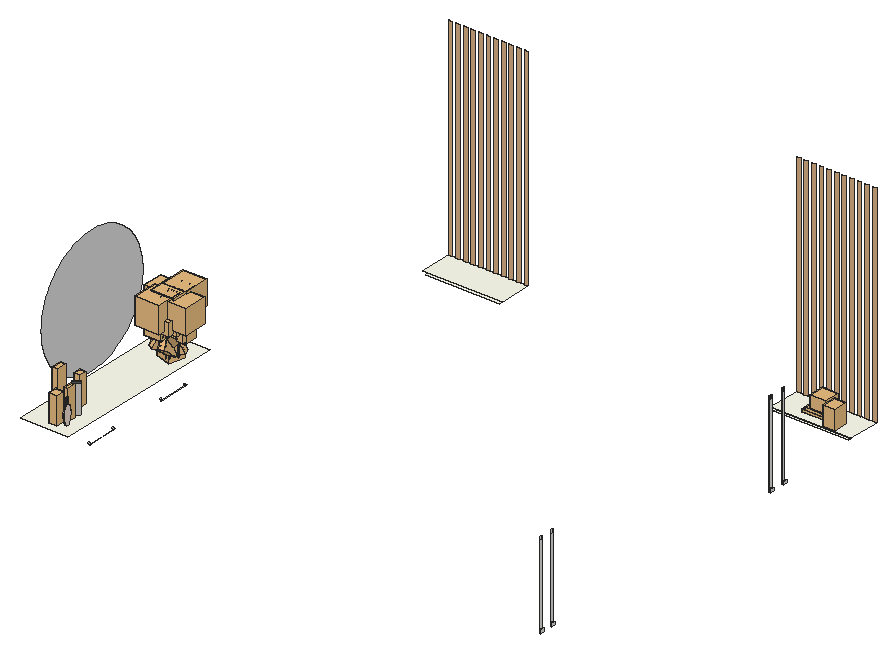
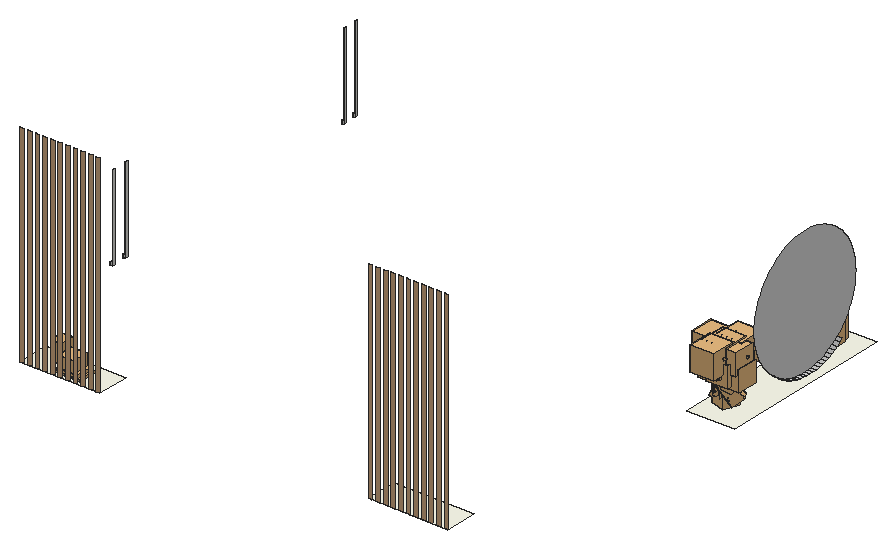
# SketchUp Ruby script. Lengths in inches.
U = 1.inch
M = Sketchup.active_model
def pt(a) = Geom::Point3d.new(a.map { |v| v * U })
def face(e, loops, mat)
  f = e.add_face(loops[0].map { |a| pt(a) })
  loops[1..].each { |l| e.add_face(l.map { |a| pt(a) }).erase! }
  f.material = f.back_material = mat if mat
  f
end
# faces: each face lists its corners as indices into pts; further lists are holes
def faces(e, pts, list, mat = nil) = list.each { |f| face(e, (f[0].is_a?(Array) ? f : [f]).map { |l| l.map { |i| pts[i] } }, mat) }
# xy, xz, yz: faces in a plane at the given z, y or x. An outline is a flat list of corners, or four numbers for a rectangle; further outlines are holes
def ring(l) = l.size == 4 ? [[l[0], l[1]], [l[2], l[1]], [l[2], l[3]], [l[0], l[3]]] : l.each_slice(2).to_a
def flat(e, list, mat, &to3) = list.each { |f| face(e, (f[0].is_a?(Array) ? f : [f]).map { |l| ring(l).map { |u, v| to3.(u, v) } }, mat) }
def xy(e, z, list, mat = nil) = flat(e, list, mat) { |x, y| [x, y, z] }
def xz(e, y, list, mat = nil) = flat(e, list, mat) { |x, z| [x, y, z] }
def yz(e, x, list, mat = nil) = flat(e, list, mat) { |y, z| [x, y, z] }
def lines(e, pts, list) = list.each { |a, b| e.add_line(pt(pts[a]), pt(pts[b])) }
# prism: a flat outline (further loops are holes) pulled along v
def prism(e, loops, v, mat = nil)
  f = face(e, loops, mat); d = Geom::Vector3d.new(v.map { |x| x * U })
  f.pushpull(f.normal.samedirection?(d) ? d.length : -d.length)
end
def box(e, o, s, mat = nil) = prism(e, [[o, [o[0] + s[0], o[1], o[2]], [o[0] + s[0], o[1] + s[1], o[2]], [o[0], o[1] + s[1], o[2]]]], [0, 0, s[2]], mat)
def at(x, y, z, deg = 0) = Geom::Transformation.translation(pt([x, y, z])) * Geom::Transformation.rotation(ORIGIN, Z_AXIS, deg.degrees)
def axes(o, x, y, z) = Geom::Transformation.new([*x, 0, *y, 0, *z, 0, *pt(o).to_a, 1])
def part(name) = M.definitions.add(name)
# library, detail: a bought-in or finely detailed component or shape, given as its bounding box
def library(name, o, s) = part(name).tap { |d| box(d.entities, o, s) }
def detail(e, o, s) = box(e.add_group.entities, o, s)
def put(e, d, t, mat = nil) = e.add_instance(d, t).tap { |i| i.material = mat if mat }
def group(e, t, mat = nil) = e.add_group.tap { |g| g.transformation = t; g.material = mat if mat }.entities
root = M.entities
M.materials.add("Guerlain-Terracotta-Le-parfum1").color = [235, 217, 205]
M.materials.add("Material \#1").color = [0, 0, 0]
M.materials["Material \#1"].alpha = 0.02
M.materials.add("Material \#2").color = [190, 173, 82]
M.materials.add("[0053_Ivory]").color = [255, 255, 240]
M.materials.add("[0135_DarkGray]").color = [81, 81, 81]
M.materials.add("[Formica Laminate Light]").color = [219, 178, 137]
M.materials.add("[Mirror 02]").color = [216, 216, 216]
M.materials.add("parfumlegacycristianoronaldo").color = [199, 196, 192]
M.materials.add("stebel1").color = [28, 33, 12]
M.materials.add("steklo zelenkovatoie1").color = [255, 255, 255]
M.materials["steklo zelenkovatoie1"].alpha = 0.01
c1 = library("_2_Bo6",[964.11,-137.96,0],[33.44,269.06,364.17])
c2 = library("Potted succulent",[-0.0625,-0.27,0],[4.39,5.31,7.09])
c3 = library("_2_Books_",[998.35,-139.66,0],[33.41,270.76,308.82])
c4 = library("Potted succulent \#1",[-0.84,-0.93,0],[5.95,6.01,4.45])
c5 = library("3DGeom~1_Defintion",[-52.13,-413.8,-261.9],[525.02,1000,523.8])
c6 = library("3DGeom~2_Defintion",[-50.59,-505.34,-385.42],[772.63,1000,770.84])
c7 = library("3DGeom~3_Defintion",[-29.0625,-449.47,-46.19],[316.66,1000,422.96])
c8 = library("3DGeom~4_Defintion",[-108.73,-466.24,-10.56],[206.74,1000,21.12])
c9 = library("3DGeom~24_Defintion",[-29.43,-617.96,-68.09],[452.88,1000,135.79])
c10 = library("3DGeom~25_Defintion",[-610.43,-341.49,-497.01],[982.35,1000,969.41])
c11 = library("3DGeom~26_Defintion",[-154.21,-582.64,-13.2],[230.85,1000,89.07])
c12 = library("3DGeom~46_Defintion",[-99.32,-628.8,-45.04],[163.52,1000,86.15])
c13 = library("3DGeom~47_Defintion",[-610.43,-341.49,-497.01],[982.35,1000,969.41])
c14 = library("3DGeom~67_Defintion",[-119.83,-464.72,-82.11],[221.96,1000,101.36])
c15 = library("3DGeom~68_Defintion",[-87.7,-569.68,-8.51],[166.72,1000,17.02])
c16 = library("3DGeom~88_Defintion",[-29.05,-445.66,-46.32],[158.62,1000,383.8])
c17 = library("3DGeom~108_Defintion",[-29.05,-445.66,-46.32],[158.62,1000,383.8])
c18 = library("3DGeom~128_Defintion",[-59.54,-603.37,-20.8],[132.36,1000,205.61])
c19 = library("3DGeom~210_Defintion",[-52.61,-408.84,-35.61],[338.09,1000,556.23])
c20 = library("3DGeom~148_Defintion",[51.2,-373.87,-225.05],[965.37,1000,237.2])
c21 = library("3DGeom~168_Defintion",[-240.01,-591.63,-7.88],[312.88,1000,313.07])
c22 = library("3DGeom~188_Defintion",[-38.1,-581.48,-8.09],[235.64,1000,465.37])
c23 = library("3DGeom~208_Defintion",[-31.71,-599.5,-29.35],[299.97,1000,62.63])
c24 = library("3DGeom~209_Defintion",[-610.43,-341.49,-497.01],[982.35,1000,969.41])
c25 = library("3DGeom~230_Defintion",[-52.27,-610.5,-175.11],[119.82,1000,194.62])
c26 = library("3DGeom~231_Defintion",[-610.43,-341.49,-497.01],[982.35,1000,969.41])
c27 = library("Group256\#1",[-71.58,-56.43,-7.72],[73.72,80.59,73.34])
c28 = library("Group263\#1",[-46.97,-31.33,7.1875],[18.81,31.79,41.38])
c29 = library("Group287\#1",[-50.75,-46.82,27.36],[89.41,99.07,85.64])
c30 = library("Group294\#1",[-14.22,-12.09,43.13],[18.22,30.92,53.79])
c31 = library("Group317\#1",[-1.3,-52.25,9.83],[15.89,17.75,44.41])
c32 = library("Group337\#1",[-31.87,-82.17,2.6],[77.56,78.87,47.75])
c33 = library("Group347\#1",[-4.2,-64.59,17.37],[101.32,89.76,91.67])
c34 = library("Group354\#1",[24.67,-31.86,36.01],[41.21,18.58,51.73])
c35 = library("Group376\#1",[-63.84,-14.97,-16.9],[80.46,73.53,76.87])
c36 = library("Group383\#1",[-36.625,8.77,7.86],[25.4,35.84,34.54])
c37 = library("Group405\#1",[-23.14,-24.51,-17.79],[74.54,78.39,80.19])
c38 = library("Group412\#1",[-0.27,0.9375,4.5],[35.66,26.25,34.25])
c39 = library("Group434\#1",[-64.79,-104.42,13.66],[92.35,97.65,97.85])
c40 = library("Group441\#1",[-31.23,-78.39,39.84],[22.43,44.95,44.17])
c41 = library("Group463\#1",[-31.71,-70.81,-2.87],[18.58,35.57,19.28])
c42 = library("Group483\#1",[-53.17,-75.45,-26.9375],[66.59,51.19,65.74])
c43 = library("Group492\#1",[-47.04,8.92,24.48],[89.7,95.5,90.68])
c44 = library("Group499\#1",[-12.74,38.04,47.38],[22.44,43.15,45.66])
c45 = library("Group521\#1",[-89.52,-29.26,29.33],[79.87,78.2,80.19])
c46 = library("Group528\#1",[-65.95,-0.45,51.63],[35.33,26.88,34.25])
c47 = library("Group552\#1",[-97.12,-35.39,-24.56],[60.39,79.79,77.7])
c48 = library("Group559\#1",[-90.25,-4.6,5.7],[42.56,22.1,20.27])
c49 = library("Group582\#1",[26.01,-59.49,-2.98],[35.51,41.53,26.85])
c50 = library("Group583\#1",[22.86,-47.74,0.4375],[40.62,39.02,47.67])
c51 = library("Group584\#1",[29.99,-24.89,-5.59],[36.3,43.55,36.22])
c52 = library("Group585\#1",[29.89,-48.04,-26.1],[42.74,35.82,45.2])
c53 = library("Group586\#1",[23.8,-29.02,1.04],[40.9,33.88,46.12])
c54 = library("Group587\#1",[32.33,-33.47,-29.58],[46.05,42.8,51.3])
c55 = library("Group589\#1",[32.61,-23.03,5.86],[38.87,7.41,11.92])
c56 = library("Group592\#1",[31.95,-24.5625,6.27],[41.61,5.99,14.68])
c57 = library("Group595\#1",[31.72,-30.92,5.77],[35.66,11.54,12.18])
c58 = library("Group598\#1",[32.89,-27.72,3.5],[41.82,8.31,12.73])
c59 = library("Group601\#1",[32.85,-23.81,2.26],[39.48,5.21,12.87])
c60 = library("Group604\#1",[32.97,-23.7,0.68],[37.46,10.79,14.46])
c61 = library("Group607\#1",[32.41,-24.57,4.01],[32.05,7.19,11.83])
c62 = part("Group250\#1")
put(c62.entities,c5,axes([-27.93,0.85,-67.89],[0.10942,-0.0328,0],[0,0,0.11423],[-0.0328,-0.10942,0]),"steklo zelenkovatoie1")
put(c62.entities,c6,axes([-27.93,0.85,-67.89],[0.06787,-0.02034,0],[0,0,0.07086],[-0.02034,-0.06787,0]),"Material \#1")
put(c62.entities,c7,axes([-15.1,-12.46,-31.32],[0.07432,0.06349,-0.05506],[0.07739,-0.02306,0.07788],[0.03275,-0.08957,-0.05907]),"stebel1")
put(c62.entities,c8,axes([-26.86,2.88,-49.92],[-0.05357,-0.102,0],[0,0,0.11521],[-0.102,0.05357,0]),"stebel1")
put(c62.entities,c9,axes([-11.34,-17.02,20.09],[-0.0063,0.12632,-0.10549],[-0.04747,0.09969,0.1222],[0.15758,0.03508,0.03259]),"stebel1")
put(c62.entities,c10,axes([-40.61,43.2,69.56],[-0.00654,0.00012,-0.00786],[-0.00561,-0.00724,0.00455],[-0.02646,0.03467,0.02255]),"Material \#2")
put(c62.entities,c11,axes([-18,-11.56,-13.53],[-0.06678,0.12751,0.0315],[0.04218,-0.01264,0.14061],[0.12438,0.07274,-0.03077]),"stebel1")
put(c62.entities,c12,axes([8.55,-18.5625,3.57],[0.16197,-0.04855,0],[0,0,0.16909],[-0.04855,-0.16197,0]),"stebel1")
put(c62.entities,c13,axes([25.0625,-17.88,85.16],[0.00739,0.00592,-0.00387],[-0.00618,0.00812,0.00061],[0.01647,0.00912,0.04534]),"Material \#2")
put(c62.entities,c14,axes([1.14,-28.05,-49.92],[0.04622,-0.10645,0],[0,0,0.11606],[-0.10645,-0.04622,0]),"stebel1")
put(c62.entities,c15,axes([22.47,-14.26,-19.22],[0.13689,-0.04103,0],[0,0,0.1429],[-0.04103,-0.13689,0]),"stebel1")
put(c62.entities,c16,axes([-4.88,-15.48,-41.05],[-0.09455,0.05151,-0.02857],[-0.00894,0.04086,0.10325],[0.05822,0.08993,-0.03055]),"stebel1")
put(c62.entities,c17,axes([-27.48,2.8,-44.87],[0.07693,0.07534,-0.02857],[0.04169,-0.00341,0.10325],[0.06895,-0.08199,-0.03055]),"stebel1")
put(c62.entities,c18,axes([3.67,-12.44,-8.08],[0.05195,-0.14507,-0.01714],[-0.05925,-0.03755,0.13826],[-0.13352,-0.03978,-0.06802]),"stebel1")
put(c62.entities,c19,axes([-3.07,-11.58,-26.29],[-0.07643,-0.04955,-0.05131],[-0.06867,0.03078,0.07257],[-0.01929,0.08676,-0.05505]),"stebel1")
put(c62.entities,c20,axes([0.18,9.9375,-12.85],[-0.02749,-0.03127,-0.07245],[-0.02127,-0.07095,0.03868],[-0.07599,0.03116,0.01538]),"stebel1")
put(c62.entities,c21,axes([-29.92,16.96,0.49],[-0.09159,0.11912,0.01982],[0.07962,0.04088,0.12231],[0.09078,0.08433,-0.08728]),"stebel1")
put(c62.entities,c22,axes([-18.25,-21.22,2.26],[-0.13551,0.04489,-0.03788],[-0.0213,0.0512,0.13688],[0.05473,0.13106,-0.0405]),"stebel1")
put(c62.entities,c23,axes([-16.76,7.75,-0.37],[0.12559,0.07073,-0.06232],[0.05784,0.02417,0.14398],[0.07444,-0.13811,-0.00672]),"stebel1")
put(c62.entities,c24,axes([23.22,32.08,68.47],[-0.00082,0.00868,-0.00535],[-0.00922,0.00166,0.00409],[0.02084,0.02475,0.03693]),"Material \#2")
put(c62.entities,c25,axes([-32.65,4.47,-9.81],[-0.14512,0.04201,-0.05532],[-0.05817,-0.00348,0.14997],[0.03797,0.15527,0.01833]),"stebel1")
put(c62.entities,c26,axes([-77.51,1.58,60.26],[-0.00529,-0.00603,-0.00635],[0.00581,-0.00796,0.00273],[-0.03144,-0.01054,0.03621]),"Material \#2")
put(c62.entities,c27,at(0,0,0))
put(c62.entities,c28,at(0,0,0))
put(c62.entities,c29,at(0,0,0))
put(c62.entities,c30,at(0,0,0))
put(c62.entities,c31,at(0,0,0))
put(c62.entities,c32,at(0,0,0))
put(c62.entities,c33,at(0,0,0))
put(c62.entities,c34,at(0,0,0))
put(c62.entities,c35,at(0,0,0))
put(c62.entities,c36,at(0,0,0))
put(c62.entities,c37,at(0,0,0))
put(c62.entities,c38,at(0,0,0))
put(c62.entities,c39,at(0,0,0))
put(c62.entities,c40,at(0,0,0))
put(c62.entities,c41,at(0,0,0))
put(c62.entities,c42,at(0,0,0))
put(c62.entities,c43,at(0,0,0))
put(c62.entities,c44,at(0,0,0))
put(c62.entities,c45,at(0,0,0))
put(c62.entities,c46,at(0,0,0))
put(c62.entities,c47,at(0,0,0))
put(c62.entities,c48,at(0,0,0))
put(c62.entities,c49,at(0,0,0))
put(c62.entities,c50,at(0,0,0))
put(c62.entities,c51,at(0,0,0))
put(c62.entities,c52,at(0,0,0))
put(c62.entities,c53,at(0,0,0))
put(c62.entities,c54,at(0,0,0))
put(c62.entities,c55,at(0,0,0))
put(c62.entities,c56,at(0,0,0))
put(c62.entities,c57,at(0,0,0))
put(c62.entities,c58,at(0,0,0))
put(c62.entities,c59,at(0,0,0))
put(c62.entities,c60,at(0,0,0))
put(c62.entities,c61,at(0,0,0))
xy(root,43.794,[[24.639,44.595,24.875,56.5],[24.639,78.595,24.875,90.5]])
xy(root,45.244,[[39.88,185,68.12,186],[171.88,185,200.12,186]],"[0053_Ivory]")
xy(root,46.244,[[38.88,185,69.12,197],[170.88,185,201.12,197]],"[0053_Ivory]")
xy(root,50.387,[[19.07,39.927,19.63,40.97]],"Guerlain-Terracotta-Le-parfum1")
xy(root,50.387,[[[6,35.11,24,102.422],[19.07,39.927,19.63,40.97]]],"[0053_Ivory]")
xy(root,50.766,[[17.077,45.58,16.024,46.893,18.094,48.815,19.146,47.503]])
xy(root,52.343,[[210,27.045,209.361,27.38,209.125,27.38,209.125,28.052,209.361,28.052,210,28.388],[210,32.232,209.361,32.568,209.125,32.568,209.125,33.239,209.361,33.239,210,33.575],[210,135.92,209.361,136.255,209.125,136.255,209.125,136.927,209.361,136.927,210,137.263],[210,141.92,209.361,142.255,209.125,142.255,209.125,142.927,209.361,142.927,210,143.263]])
xy(root,53.603,[[210,27.045,210,28.388,209.361,28.052,209.361,27.38],[210,32.232,210,33.575,209.361,33.239,209.361,32.568],[210,135.92,210,137.263,209.361,136.927,209.361,136.255],[210,141.92,210,143.263,209.361,142.927,209.361,142.255]])
xy(root,57.471,[[19.045,40.163,19.649,40.792]],"Guerlain-Terracotta-Le-parfum1")
xy(root,57.984,[[19.353,40.0625,19.254,40.077,19.161,40.118,19.082,40.184,19.021,40.269,18.982,40.369,18.969,40.476,18.982,40.583,19.021,40.682,19.082,40.768,19.161,40.833,19.254,40.875,19.353,40.889,19.452,40.875,19.545,40.833,19.624,40.768,19.685,40.682,19.724,40.583,19.737,40.476,19.724,40.369,19.685,40.269,19.624,40.184,19.545,40.118,19.452,40.077]])
xy(root,59.52,[[19.353,40.0625,19.452,40.077,19.545,40.118,19.624,40.184,19.685,40.269,19.724,40.369,19.737,40.476,19.724,40.583,19.685,40.682,19.624,40.768,19.545,40.833,19.452,40.875,19.353,40.889,19.254,40.875,19.161,40.833,19.082,40.768,19.021,40.682,18.982,40.583,18.969,40.476,18.982,40.369,19.021,40.269,19.082,40.184,19.161,40.118,19.254,40.077]],"[0135_DarkGray]")
xy(root,61.174,[[17.077,45.58,19.146,47.503,18.094,48.815,16.024,46.893]],"[0135_DarkGray]")
xz(root,27.38,[[209.125,52.343,209.361,84.893]])
xz(root,28.052,[[209.125,52.343,209.361,84.893]])
xz(root,32.568,[[209.125,52.343,209.361,84.893]])
xz(root,33.239,[[209.125,52.343,209.361,84.893]])
xz(root,40.156,[[19.045,57.429,19.649,57.436],[19.045,57.436,19.649,57.443]],"Guerlain-Terracotta-Le-parfum1")
xz(root,136.255,[[209.125,52.343,209.361,84.893]])
xz(root,136.927,[[209.125,52.343,209.361,84.893]])
xz(root,142.255,[[209.125,52.343,209.361,84.893]])
xz(root,142.927,[[209.125,52.343,209.361,84.893]])
xz(root,197,[[38.88,46.244,40.32,126],[41.76,46.244,43.2,126],[44.64,46.244,46.08,126],[47.52,46.244,48.96,126],[50.4,46.244,51.84,126],
  [53.28,46.244,54.72,126],[56.16,46.244,57.6,126],[59.04,46.244,60.48,126],[61.92,46.244,63.36,126],[64.8,46.244,66.24,126],
  [67.68,46.244,69.12,126],[170.88,46.244,172.32,126],[173.76,46.244,175.2,126],[176.64,46.244,178.08,126],[179.52,46.244,180.96,126],
  [182.4,46.244,183.84,126],[185.28,46.244,186.72,126],[188.16,46.244,189.6,126],[191.04,46.244,192.48,126],[193.92,46.244,195.36,126],
  [196.8,46.244,198.24,126],[199.68,46.244,201.12,126]],"[Formica Laminate Light]")
yz(root,8,[[66.545,53.326,68.052,53.373,69.553,53.515,71.042,53.751,72.513,54.08,73.961,54.5,75.38,55.011,76.763,55.61,78.107,56.294,79.404,57.062,80.651,57.909,81.843,58.833,82.974,59.831,84.04,60.897,85.037,62.028,85.961,63.219,86.808,64.466,87.576,65.764,88.26,67.107,88.859,68.491,89.37,69.909,89.791,71.357,90.119,72.829,90.355,74.318,90.497,75.819,90.545,77.326,90.497,78.833,90.355,80.334,90.119,81.823,89.791,83.294,89.37,84.742,88.859,86.161,88.26,87.545,87.576,88.888,86.808,90.186,85.961,91.433,85.037,92.624,84.04,93.755,82.974,94.821,81.843,95.818,80.651,96.742,79.404,97.59,78.107,98.357,76.763,99.042,75.38,99.64,73.961,100.151,72.513,100.572,71.042,100.901,69.553,101.137,68.052,101.278,66.545,101.326,65.038,101.278,63.537,101.137,62.047,100.901,60.576,100.572,59.128,100.151,57.71,99.64,56.326,99.042,54.982,98.357,53.685,97.59,52.4375,96.742,51.246,95.818,50.115,94.821,49.049,93.755,48.052,92.624,47.128,91.433,46.281,90.186,45.513,88.888,44.829,87.545,44.23,86.161,43.719,84.742,43.299,83.294,42.97,81.823,42.734,80.334,42.592,78.833,42.545,77.326,42.592,75.819,42.734,74.318,42.97,72.829,43.299,71.357,43.719,69.909,44.23,68.491,44.829,67.107,45.513,65.764,46.281,64.466,47.128,63.219,48.052,62.028,49.049,60.897,50.115,59.831,51.246,58.833,52.4375,57.909,53.685,57.062,54.982,56.294,56.326,55.61,57.71,55.011,59.128,54.5,60.576,54.08,62.047,53.751,63.537,53.515,65.038,53.373]],"[Mirror 02]")
yz(root,19.045,[[40.163,57.4,40.161,57.404,40.159,57.41,40.158,57.415,40.156,57.429,40.156,57.443,40.157,57.449,40.158,57.456,40.159,57.462,40.161,57.467,40.163,57.471,40.792,57.471,40.795,57.47,40.798,57.466,40.801,57.461,40.803,57.454,40.804,57.445,40.805,57.437,40.803,57.419,40.801,57.412,40.798,57.407,40.795,57.403]],"Guerlain-Terracotta-Le-parfum1")
yz(root,19.07,[[39.927,50.387,39.693,50.727,39.471,51.233,39.294,51.85,39.169,52.553,39.102,53.309,39.095,54.087,39.149,54.851,39.261,55.569,39.427,56.208,39.639,56.741,39.888,57.144,40.163,57.4,40.795,57.403,41.068,57.141,41.315,56.731,41.524,56.193,41.687,55.55,41.795,54.83,41.845,54.066,41.834,53.291,41.762,52.54,41.633,51.845,41.452,51.237,41.228,50.744,40.97,50.387]],"Guerlain-Terracotta-Le-parfum1")
yz(root,19.63,[[39.927,50.387,40.97,50.387,41.228,50.744,41.452,51.237,41.633,51.845,41.762,52.54,41.834,53.291,41.845,54.066,41.795,54.83,41.687,55.55,41.524,56.193,41.315,56.731,41.068,57.141,40.795,57.403,40.163,57.4,39.888,57.144,39.639,56.741,39.427,56.208,39.261,55.569,39.149,54.851,39.095,54.087,39.102,53.309,39.169,52.553,39.294,51.85,39.471,51.233,39.693,50.727]],"Guerlain-Terracotta-Le-parfum1")
yz(root,19.649,[[40.163,57.4,40.795,57.403,40.798,57.407,40.801,57.412,40.803,57.419,40.805,57.437,40.804,57.445,40.803,57.454,40.801,57.461,40.798,57.466,40.795,57.47,40.792,57.471,40.163,57.471,40.161,57.467,40.159,57.462,40.158,57.456,40.157,57.449,40.156,57.443,40.156,57.429,40.158,57.415,40.159,57.41,40.161,57.404]],"Guerlain-Terracotta-Le-parfum1")
yz(root,209.125,[[27.38,52.343,28.052,84.893],[32.568,52.343,33.239,84.893],[136.255,52.343,136.927,84.893],[142.255,52.343,142.927,84.893]])
yz(root,209.361,[[27.38,53.603,28.052,83.633],[32.568,53.603,33.239,83.633],[136.255,53.603,136.927,83.633],[142.255,53.603,142.927,83.633]])
yz(root,210,[[27.045,52.343,28.388,53.603],[32.232,52.343,33.575,53.603],[135.92,52.343,137.263,53.603],[141.92,52.343,143.263,53.603]])
p = [[24,44.595,44.13],[24.639,44.595,43.794],[24.639,45.056,43.794],[24,45.056,44.13],[24,56.5,44.13],[24.639,56.5,43.794],
  [24.639,56.039,43.794],[24,56.039,44.13],[24,78.595,44.13],[24.639,78.595,43.794],[24.639,79.056,43.794],[24,79.056,44.13],
  [24,90.5,44.13],[24.639,90.5,43.794],[24.639,90.039,43.794],[24,90.039,44.13],[19.07,39.927,50.387],[19.63,39.927,50.387],
  [19.63,39.693,50.727],[19.07,39.693,50.727],[19.07,41.228,50.744],[19.63,41.228,50.744],[19.63,40.97,50.387],[19.07,40.97,50.387],
  [19.63,39.471,51.233],[19.07,39.471,51.233],[19.07,41.452,51.237],[19.63,41.452,51.237],[16.024,46.893,50.766],[17.077,45.58,50.766],
  [17.077,45.58,61.174],[16.024,46.893,61.174],[19.146,47.503,50.766],[19.146,47.503,61.174],[18.094,48.815,61.174],[18.094,48.815,50.766],
  [19.63,39.294,51.85],[19.07,39.294,51.85],[19.07,41.633,51.845],[19.63,41.633,51.845],[19.07,41.762,52.54],[19.63,41.762,52.54],
  [19.63,39.169,52.553],[19.07,39.169,52.553],[210,27.045,52.343],[209.361,27.38,52.343],[209.361,27.38,53.603],[210,27.045,53.603],
  [209.361,28.052,53.603],[210,28.388,53.603],[210,28.388,52.343],[209.361,28.052,52.343],[210,32.232,52.343],[209.361,32.568,52.343],
  [209.361,32.568,53.603],[210,32.232,53.603],[209.361,33.239,53.603],[210,33.575,53.603],[210,33.575,52.343],[209.361,33.239,52.343],
  [210,135.92,52.343],[209.361,136.255,52.343],[209.361,136.255,53.603],[210,135.92,53.603],[209.361,136.927,53.603],[210,137.263,53.603],
  [210,137.263,52.343],[209.361,136.927,52.343],[210,141.92,52.343],[209.361,142.255,52.343],[209.361,142.255,53.603],[210,141.92,53.603],
  [209.361,142.927,53.603],[210,143.263,53.603],[210,143.263,52.343],[209.361,142.927,52.343],[19.07,41.834,53.291],[19.63,41.834,53.291],
  [19.63,39.102,53.309],[19.07,39.102,53.309],[19.63,39.095,54.087],[19.07,39.095,54.087],[19.07,41.845,54.066],[19.63,41.845,54.066],
  [6,65.038,53.373],[6,66.545,53.326],[8,66.545,53.326],[8,65.038,53.373],[6,68.052,53.373],[8,68.052,53.373],
  [6,63.537,53.515],[8,63.537,53.515],[6,69.553,53.515],[8,69.553,53.515],[6,62.047,53.751],[8,62.047,53.751],
  [6,71.042,53.751],[8,71.042,53.751],[6,60.576,54.08],[8,60.576,54.08],[6,72.513,54.08],[8,72.513,54.08],
  [19.63,39.149,54.851],[19.07,39.149,54.851],[19.07,41.795,54.83],[19.63,41.795,54.83],[6,59.128,54.5],[8,59.128,54.5],
  [6,73.961,54.5],[8,73.961,54.5],[6,57.71,55.011],[8,57.71,55.011],[6,75.38,55.011],[8,75.38,55.011],
  [19.07,41.687,55.55],[19.63,41.687,55.55],[19.63,39.261,55.569],[19.07,39.261,55.569],[6,56.326,55.61],[8,56.326,55.61],
  [6,76.763,55.61],[8,76.763,55.61],[19.07,41.524,56.193],[19.63,41.524,56.193],[19.63,39.427,56.208],[19.07,39.427,56.208],
  [6,54.982,56.294],[8,54.982,56.294],[6,78.107,56.294],[8,78.107,56.294],[19.63,39.639,56.741],[19.07,39.639,56.741],
  [19.07,41.315,56.731],[19.63,41.315,56.731],[6,53.685,57.062],[8,53.685,57.062],[6,79.404,57.062],[8,79.404,57.062],
  [19.63,39.888,57.144],[19.07,39.888,57.144],[19.07,41.068,57.141],[19.63,41.068,57.141],[19.63,40.163,57.4],[19.07,40.163,57.4],
  [19.07,40.795,57.403],[19.63,40.795,57.403],[6,52.4375,57.909],[8,52.4375,57.909],[6,80.651,57.909],[8,80.651,57.909],
  [19.045,40.163,57.4],[19.045,40.795,57.403],[19.649,40.163,57.4],[19.649,40.161,57.404],[19.045,40.161,57.404],[19.649,40.159,57.41],
  [19.045,40.159,57.41],[19.649,40.158,57.415],[19.045,40.158,57.415],[19.649,40.157,57.422],[19.045,40.157,57.422],[19.649,40.156,57.429],
  [19.045,40.156,57.429],[19.045,40.156,57.443],[19.649,40.156,57.443],[19.649,40.157,57.449],[19.045,40.157,57.449],[19.649,40.158,57.456],
  [19.045,40.158,57.456],[19.206,40.219,57.984],[19.149,40.266,57.984],[19.149,40.266,57.444],[19.206,40.219,57.444],[19.273,40.19,57.984],
  [19.273,40.19,57.444],[19.344,40.18,57.984],[19.344,40.18,57.444],[19.415,40.19,57.984],[19.415,40.19,57.444],[19.482,40.219,57.984],
  [19.482,40.219,57.444],[19.539,40.266,57.984],[19.539,40.266,57.444],[19.649,40.795,57.403],[19.105,40.328,57.984],[19.078,40.399,57.984],
  [19.078,40.399,57.444],[19.105,40.328,57.444],[19.582,40.328,57.984],[19.582,40.328,57.444],[19.61,40.399,57.984],[19.61,40.399,57.444],
  [19.068,40.476,57.984],[19.068,40.476,57.444],[19.619,40.476,57.984],[19.619,40.476,57.444],[19.078,40.553,57.984],[19.078,40.553,57.444],
  [19.61,40.553,57.984],[19.61,40.553,57.444],[19.105,40.624,57.984],[19.105,40.624,57.444],[19.149,40.686,57.984],[19.149,40.686,57.444],
  [19.539,40.686,57.984],[19.582,40.624,57.984],[19.582,40.624,57.444],[19.539,40.686,57.444],[19.206,40.733,57.984],[19.206,40.733,57.444],
  [19.273,40.762,57.984],[19.273,40.762,57.444],[19.415,40.762,57.984],[19.482,40.733,57.984],[19.482,40.733,57.444],[19.415,40.762,57.444],
  [19.045,40.798,57.407],[19.649,40.798,57.407],[19.045,40.801,57.412],[19.649,40.801,57.412],[19.045,40.803,57.419],[19.649,40.803,57.419],
  [19.045,40.804,57.428],[19.649,40.804,57.428],[19.045,40.805,57.437],[19.649,40.805,57.437],[19.045,40.804,57.445],[19.649,40.804,57.445],
  [19.045,40.803,57.454],[19.649,40.803,57.454],[19.344,40.772,57.984],[19.344,40.772,57.444],[19.649,40.159,57.462],[19.045,40.159,57.462],
  [19.649,40.161,57.467],[19.045,40.161,57.467],[19.649,40.163,57.471],[19.045,40.163,57.471],[19.045,40.801,57.461],[19.649,40.801,57.461],
  [19.045,40.798,57.466],[19.649,40.798,57.466],[19.045,40.795,57.47],[19.649,40.795,57.47],[19.045,40.792,57.471],[19.649,40.792,57.471],
  [6,51.246,58.833],[8,51.246,58.833],[6,81.843,58.833],[8,81.843,58.833],[19.161,40.118,59.52],[19.082,40.184,59.52],
  [19.082,40.184,57.984],[19.161,40.118,57.984],[19.254,40.077,59.52],[19.254,40.077,57.984],[19.353,40.0625,59.52],[19.353,40.0625,57.984],
  [19.452,40.077,59.52],[19.452,40.077,57.984],[19.545,40.118,59.52],[19.545,40.118,57.984],[19.624,40.184,59.52],[19.624,40.184,57.984],
  [19.021,40.269,59.52],[19.021,40.269,57.984],[19.685,40.269,59.52],[19.685,40.269,57.984],[18.982,40.369,59.52],[18.982,40.369,57.984],
  [19.724,40.369,59.52],[19.724,40.369,57.984],[18.969,40.476,59.52],[18.969,40.476,57.984],[19.737,40.476,59.52],[19.737,40.476,57.984],
  [18.982,40.583,59.52],[18.982,40.583,57.984],[19.724,40.583,59.52],[19.724,40.583,57.984],[19.021,40.682,59.52],[19.021,40.682,57.984],
  [19.685,40.682,59.52],[19.685,40.682,57.984],[19.082,40.768,59.52],[19.082,40.768,57.984],[19.624,40.768,59.52],[19.624,40.768,57.984],
  [19.161,40.833,59.52],[19.161,40.833,57.984],[19.254,40.875,59.52],[19.254,40.875,57.984],[19.452,40.875,59.52],[19.545,40.833,59.52],
  [19.545,40.833,57.984],[19.452,40.875,57.984],[19.353,40.889,59.52],[19.353,40.889,57.984],[19.678,89.759,51.324],[20.678,89.759,51.324],
  [20.678,90.759,51.324]]
faces(root,p,[[0,1,2,3],[4,5,6,7],[8,9,10,11],[12,13,14,15],[44,45,46,47],[48,49,50,51],[52,53,54,55],[56,57,58,59],
  [60,61,62,63],[64,65,66,67],[68,69,70,71],[72,73,74,75],[144,143,142,145]])
faces(root,p,[[16,17,18,19],[20,21,22,23],[19,18,24,25],[26,27,21,20],[25,24,36,37],[38,39,27,26],[40,41,39,38],[37,36,42,43],
  [76,77,41,40],[43,42,78,79],[79,78,80,81],[82,83,77,76],[81,80,102,103],[104,105,83,82],[114,115,105,104],[103,102,116,117],
  [122,123,115,114],[117,116,124,125],[125,124,130,131],[132,133,123,122],[131,130,138,139],[140,141,133,132],[139,138,142,143],[144,145,141,140],
  [144,143,150,151],[143,142,152,153,154,150],[154,153,155,156],[156,155,157,158],[158,157,159,160],[160,159,161,162],[163,164,165,166],[166,165,167,168],
  [169,170,171,172],[173,169,172,174],[175,173,174,176],[177,175,176,178],[179,177,178,180],[181,179,180,182],[142,145,183,152],[184,185,186,187],
  [170,184,187,171],[188,181,182,189],[190,188,189,191],[185,192,193,186],[194,190,191,195],[192,196,197,193],[198,194,195,199],[196,200,201,197],
  [200,202,203,201],[204,205,206,207],[205,198,199,206],[202,208,209,203],[208,210,211,209],[212,213,214,215],[213,204,207,214],[216,217,183,145,144,151],
  [218,219,217,216],[220,221,219,218],[222,223,221,220],[224,225,223,222],[226,227,225,224],[228,229,227,226],[230,212,215,231],[210,230,231,211],
  [168,167,232,233],[233,232,234,235],[235,234,236,237],[238,239,229,228],[240,241,239,238],[242,243,241,240],[244,245,243,242],[250,251,252,253],
  [254,250,253,255],[256,254,255,257],[258,256,257,259],[260,258,259,261],[262,260,261,263],[251,264,265,252],[266,262,263,267],[264,268,269,265],
  [270,266,267,271],[268,272,273,269],[274,270,271,275],[272,276,277,273],[278,274,275,279],[276,280,281,277],[282,278,279,283],[280,284,285,281],
  [286,282,283,287],[284,288,289,285],[288,290,291,289],[292,293,294,295],[293,286,287,294],[290,296,297,291],[296,292,295,297]],"Guerlain-Terracotta-Le-parfum1")
faces(root,p,[[28,29,30,31],[32,33,30,29],[28,31,34,35],[32,35,34,33]],"parfumlegacycristianoronaldo")
faces(root,p,[[84,85,86,87],[85,88,89,86],[90,84,87,91],[88,92,93,89],[94,90,91,95],[92,96,97,93],[98,94,95,99],[96,100,101,97],
  [106,98,99,107],[100,108,109,101],[110,106,107,111],[108,112,113,109],[118,110,111,119],[112,120,121,113],[126,118,119,127],[120,128,129,121],
  [134,126,127,135],[128,136,137,129],[146,134,135,147],[136,148,149,137],[246,146,147,247],[148,248,249,149]],"[Mirror 02]")
lines(root,p,[[298,299],[299,300],[300,298]])
detail(root,[14.15,38.25,50.19],[3.09,3.31,10.3])
detail(root,[17.55,41.48,50.74],[1.22,3.28,11.37])
detail(root,[12.76,41.74,50.87],[2.13,4.06,16.28])
detail(root,[14.57,49.85,51.35],[2.39,2.7,10.93])
put(root,c1,axes([179.68,191.98,21.17],[0,0,0.02601],[0,-0.02601,0],[0.02601,0,0]))
put(root,c2,at(190.19,185.81,46.29))
put(root,c3,axes([180.625,191.98,21.17],[0,0,0.02601],[0,-0.02601,0],[0.02601,0,0]))
put(root,c4,at(183.03,189.99,48))
put(root,c62,axes([18.16,92.59,61.91],[0.1,0,0],[0,0.1,0],[0,0,0.1]))
